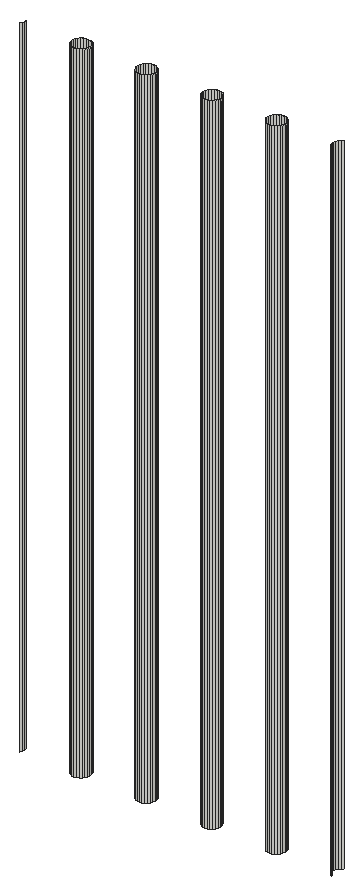
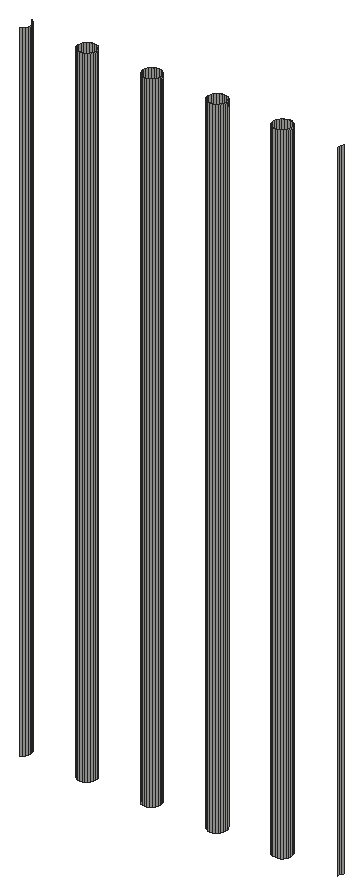
# SketchUp Ruby script. Lengths in inches.
U = 1.inch
M = Sketchup.active_model
def pt(a) = Geom::Point3d.new(a.map { |v| v * U })
def face(e, loops, mat)
  f = e.add_face(loops[0].map { |a| pt(a) })
  loops[1..].each { |l| e.add_face(l.map { |a| pt(a) }).erase! }
  f.material = f.back_material = mat if mat
  f
end
# faces: each face lists its corners as indices into pts; further lists are holes
def faces(e, pts, list, mat = nil) = list.each { |f| face(e, (f[0].is_a?(Array) ? f : [f]).map { |l| l.map { |i| pts[i] } }, mat) }
# xy, xz, yz: faces in a plane at the given z, y or x. An outline is a flat list of corners, or four numbers for a rectangle; further outlines are holes
def ring(l) = l.size == 4 ? [[l[0], l[1]], [l[2], l[1]], [l[2], l[3]], [l[0], l[3]]] : l.each_slice(2).to_a
def flat(e, list, mat, &to3) = list.each { |f| face(e, (f[0].is_a?(Array) ? f : [f]).map { |l| ring(l).map { |u, v| to3.(u, v) } }, mat) }
def xy(e, z, list, mat = nil) = flat(e, list, mat) { |x, y| [x, y, z] }
def xz(e, y, list, mat = nil) = flat(e, list, mat) { |x, z| [x, y, z] }
def yz(e, x, list, mat = nil) = flat(e, list, mat) { |y, z| [x, y, z] }
def lines(e, pts, list) = list.each { |a, b| e.add_line(pt(pts[a]), pt(pts[b])) }
# prism: a flat outline (further loops are holes) pulled along v
def prism(e, loops, v, mat = nil)
  f = face(e, loops, mat); d = Geom::Vector3d.new(v.map { |x| x * U })
  f.pushpull(f.normal.samedirection?(d) ? d.length : -d.length)
end
def box(e, o, s, mat = nil) = prism(e, [[o, [o[0] + s[0], o[1], o[2]], [o[0] + s[0], o[1] + s[1], o[2]], [o[0], o[1] + s[1], o[2]]]], [0, 0, s[2]], mat)
def at(x, y, z, deg = 0) = Geom::Transformation.translation(pt([x, y, z])) * Geom::Transformation.rotation(ORIGIN, Z_AXIS, deg.degrees)
def axes(o, x, y, z) = Geom::Transformation.new([*x, 0, *y, 0, *z, 0, *pt(o).to_a, 1])
def part(name) = M.definitions.add(name)
# library, detail: a bought-in or finely detailed component or shape, given as its bounding box
def library(name, o, s) = part(name).tap { |d| box(d.entities, o, s) }
def detail(e, o, s) = box(e.add_group.entities, o, s)
def put(e, d, t, mat = nil) = e.add_instance(d, t).tap { |i| i.material = mat if mat }
def group(e, t, mat = nil) = e.add_group.tap { |g| g.transformation = t; g.material = mat if mat }.entities
root = M.entities
xy(root,204.9375,[[448.33,135.31,448.12,135.34,447.92,135.42,447.75,135.55,447.625,135.72,447.54,135.91,447.52,136.12,447.54,136.33,447.625,136.53,447.75,136.7,447.92,136.83,448.12,136.91,448.33,136.93,448.54,136.91,448.74,136.83,448.9,136.7,449.03,136.53,449.11,136.33,449.14,136.12,449.11,135.91,449.03,135.72,448.9,135.55,448.74,135.42,448.54,135.34],[454.33,135.31,454.12,135.34,453.92,135.42,453.75,135.55,453.625,135.72,453.54,135.91,453.52,136.12,453.54,136.33,453.625,136.53,453.75,136.7,453.92,136.83,454.12,136.91,454.33,136.93,454.54,136.91,454.74,136.83,454.9,136.7,455.03,136.53,455.11,136.33,455.14,136.12,455.11,135.91,455.03,135.72,454.9,135.55,454.74,135.42,454.54,135.34],[460.33,135.31,460.12,135.34,459.92,135.42,459.75,135.55,459.625,135.72,459.54,135.91,459.52,136.12,459.54,136.33,459.625,136.53,459.75,136.7,459.92,136.83,460.12,136.91,460.33,136.93,460.54,136.91,460.74,136.83,460.9,136.7,461.03,136.53,461.11,136.33,461.14,136.12,461.11,135.91,461.03,135.72,460.9,135.55,460.74,135.42,460.54,135.34],[466.27,135.31,466.06,135.34,465.86,135.42,465.69,135.55,465.5625,135.72,465.48,135.91,465.45,136.12,465.48,136.33,465.5625,136.53,465.69,136.7,465.86,136.83,466.06,136.91,466.27,136.93,466.48,136.91,466.67,136.83,466.84,136.7,466.97,136.53,467.05,136.33,467.08,136.12,467.05,135.91,466.97,135.72,466.84,135.55,466.67,135.42,466.48,135.34]])
p = [[447.92,135.42,204.9375],[448.12,135.34,204.9375],[448.12,135.34,264.83],[447.92,135.42,264.83],[448.33,135.31,204.9375],[448.33,135.31,264.83],
  [448.54,135.34,204.9375],[448.54,135.34,264.83],[448.74,135.42,204.9375],[448.74,135.42,264.83],[453.92,135.42,204.9375],[454.12,135.34,204.9375],
  [454.12,135.34,264.83],[453.92,135.42,264.83],[454.33,135.31,204.9375],[454.33,135.31,264.83],[454.54,135.34,204.9375],[454.54,135.34,264.83],
  [454.74,135.42,204.9375],[454.74,135.42,264.83],[459.92,135.42,204.9375],[460.12,135.34,204.9375],[460.12,135.34,264.83],[459.92,135.42,264.83],
  [460.33,135.31,204.9375],[460.33,135.31,264.83],[460.54,135.34,204.9375],[460.54,135.34,264.83],[460.74,135.42,204.9375],[460.74,135.42,264.83],
  [465.86,135.42,204.9375],[466.06,135.34,204.9375],[466.06,135.34,264.83],[465.86,135.42,264.83],[466.27,135.31,204.9375],[466.27,135.31,264.83],
  [466.48,135.34,204.9375],[466.48,135.34,264.83],[466.67,135.42,204.9375],[466.67,135.42,264.83],[447.75,135.55,204.9375],[447.75,135.55,264.83],
  [448.9,135.55,204.9375],[448.9,135.55,264.83],[453.75,135.55,204.9375],[453.75,135.55,264.83],[454.9,135.55,204.9375],[454.9,135.55,264.83],
  [459.75,135.55,204.9375],[459.75,135.55,264.83],[460.9,135.55,204.9375],[460.9,135.55,264.83],[465.69,135.55,204.9375],[465.69,135.55,264.83],
  [466.84,135.55,204.9375],[466.84,135.55,264.83],[471.69,135.55,204.9375],[471.86,135.42,204.9375],[471.86,135.42,264.83],[471.69,135.55,264.83],
  [447.625,135.72,204.9375],[447.625,135.72,264.83],[449.03,135.72,204.9375],[449.03,135.72,264.83],[453.625,135.72,204.9375],[453.625,135.72,264.83],
  [455.03,135.72,204.9375],[455.03,135.72,264.83],[459.625,135.72,204.9375],[459.625,135.72,264.83],[461.03,135.72,204.9375],[461.03,135.72,264.83],
  [465.5625,135.72,204.9375],[465.5625,135.72,264.83],[466.97,135.72,204.9375],[466.97,135.72,264.83],[471.5625,135.72,204.9375],[471.5625,135.72,264.83],
  [443.03,135.72,204.9375],[443.11,135.91,204.9375],[443.11,135.91,264.83],[443.03,135.72,264.83],[447.54,135.91,204.9375],[447.54,135.91,264.83],
  [449.11,135.91,204.9375],[449.11,135.91,264.83],[453.54,135.91,204.9375],[453.54,135.91,264.83],[455.11,135.91,204.9375],[455.11,135.91,264.83],
  [459.54,135.91,204.9375],[459.54,135.91,264.83],[461.11,135.91,204.9375],[461.11,135.91,264.83],[465.48,135.91,204.9375],[465.48,135.91,264.83],
  [467.05,135.91,204.9375],[467.05,135.91,264.83],[471.48,135.91,204.9375],[471.48,135.91,264.83],[443.14,136.12,204.9375],[443.14,136.12,264.83],
  [447.52,136.12,204.9375],[447.52,136.12,264.83],[449.14,136.12,204.9375],[449.14,136.12,264.83],[453.52,136.12,204.9375],[453.52,136.12,264.83],
  [455.14,136.12,204.9375],[455.14,136.12,264.83],[459.52,136.12,204.9375],[459.52,136.12,264.83],[461.14,136.12,204.9375],[461.14,136.12,264.83],
  [465.45,136.12,204.9375],[465.45,136.12,264.83],[467.08,136.12,204.9375],[467.08,136.12,264.83],[471.45,136.12,204.9375],[471.45,136.12,264.83],
  [443.11,136.33,204.9375],[443.11,136.33,264.83],[447.54,136.33,204.9375],[447.54,136.33,264.83],[449.11,136.33,204.9375],[449.11,136.33,264.83],
  [453.54,136.33,204.9375],[453.54,136.33,264.83],[455.11,136.33,204.9375],[455.11,136.33,264.83],[459.54,136.33,204.9375],[459.54,136.33,264.83],
  [461.11,136.33,204.9375],[461.11,136.33,264.83],[465.48,136.33,204.9375],[465.48,136.33,264.83],[467.05,136.33,204.9375],[467.05,136.33,264.83],
  [471.48,136.33,204.9375],[471.48,136.33,264.83],[447.625,136.53,204.9375],[447.625,136.53,264.83],[449.03,136.53,204.9375],[449.03,136.53,264.83],
  [453.625,136.53,204.9375],[453.625,136.53,264.83],[455.03,136.53,204.9375],[455.03,136.53,264.83],[459.625,136.53,204.9375],[459.625,136.53,264.83],
  [461.03,136.53,204.9375],[461.03,136.53,264.83],[465.5625,136.53,204.9375],[465.5625,136.53,264.83],[466.97,136.53,204.9375],[466.97,136.53,264.83],
  [471.5625,136.53,204.9375],[471.5625,136.53,264.83],[447.75,136.7,204.9375],[447.75,136.7,264.83],[448.9,136.7,204.9375],[448.9,136.7,264.83],
  [453.75,136.7,204.9375],[453.75,136.7,264.83],[454.9,136.7,204.9375],[454.9,136.7,264.83],[459.75,136.7,204.9375],[459.75,136.7,264.83],
  [460.9,136.7,204.9375],[460.9,136.7,264.83],[465.69,136.7,204.9375],[465.69,136.7,264.83],[466.84,136.7,204.9375],[466.84,136.7,264.83],
  [471.69,136.7,204.9375],[471.69,136.7,264.83],[447.92,136.83,204.9375],[447.92,136.83,264.83],[448.74,136.83,204.9375],[448.74,136.83,264.83],
  [453.92,136.83,204.9375],[453.92,136.83,264.83],[454.74,136.83,204.9375],[454.74,136.83,264.83],[459.92,136.83,204.9375],[459.92,136.83,264.83],
  [460.74,136.83,204.9375],[460.74,136.83,264.83],[465.86,136.83,204.9375],[465.86,136.83,264.83],[466.67,136.83,204.9375],[466.67,136.83,264.83],
  [471.86,136.83,204.9375],[471.86,136.83,264.83],[448.12,136.91,204.9375],[448.12,136.91,264.83],[448.54,136.91,204.9375],[448.54,136.91,264.83],
  [454.12,136.91,204.9375],[454.12,136.91,264.83],[454.54,136.91,204.9375],[454.54,136.91,264.83],[460.12,136.91,204.9375],[460.12,136.91,264.83],
  [460.54,136.91,204.9375],[460.54,136.91,264.83],[466.06,136.91,204.9375],[466.06,136.91,264.83],[466.48,136.91,204.9375],[466.48,136.91,264.83],
  [448.33,136.93,204.9375],[448.33,136.93,264.83],[454.33,136.93,204.9375],[454.33,136.93,264.83],[460.33,136.93,204.9375],[460.33,136.93,264.83],
  [466.27,136.93,204.9375],[466.27,136.93,264.83],[466.27,136.12,264.83],[466.27,136.12,204.9375],[460.27,136.12,264.83],[460.27,136.12,204.9375],
  [454.27,136.12,264.83],[454.27,136.12,204.9375],[448.27,136.12,264.83],[448.27,136.12,204.9375]]
faces(root,p,[[0,1,2,3],[1,4,5,2],[4,6,7,5],[6,8,9,7],[10,11,12,13],[11,14,15,12],[14,16,17,15],[16,18,19,17],
  [20,21,22,23],[21,24,25,22],[24,26,27,25],[26,28,29,27],[30,31,32,33],[31,34,35,32],[34,36,37,35],[36,38,39,37],
  [40,0,3,41],[8,42,43,9],[44,10,13,45],[18,46,47,19],[48,20,23,49],[28,50,51,29],[52,30,33,53],[38,54,55,39],
  [56,57,58,59],[60,40,41,61],[42,62,63,43],[64,44,45,65],[46,66,67,47],[68,48,49,69],[50,70,71,51],[72,52,53,73],
  [54,74,75,55],[76,56,59,77],[78,79,80,81],[82,60,61,83],[62,84,85,63],[86,64,65,87],[66,88,89,67],[90,68,69,91],
  [70,92,93,71],[94,72,73,95],[74,96,97,75],[98,76,77,99],[79,100,101,80],[102,82,83,103],[84,104,105,85],[106,86,87,107],
  [88,108,109,89],[110,90,91,111],[92,112,113,93],[114,94,95,115],[96,116,117,97],[118,98,99,119],[100,120,121,101],[122,102,103,123],
  [104,124,125,105],[126,106,107,127],[108,128,129,109],[130,110,111,131],[112,132,133,113],[134,114,115,135],[116,136,137,117],[138,118,119,139],
  [140,122,123,141],[124,142,143,125],[144,126,127,145],[128,146,147,129],[148,130,131,149],[132,150,151,133],[152,134,135,153],[136,154,155,137],
  [156,138,139,157],[158,140,141,159],[142,160,161,143],[162,144,145,163],[146,164,165,147],[166,148,149,167],[150,168,169,151],[170,152,153,171],
  [154,172,173,155],[174,156,157,175],[176,158,159,177],[160,178,179,161],[180,162,163,181],[164,182,183,165],[184,166,167,185],[168,186,187,169],
  [188,170,171,189],[172,190,191,173],[192,174,175,193],[194,176,177,195],[178,196,197,179],[198,180,181,199],[182,200,201,183],[202,184,185,203],
  [186,204,205,187],[206,188,189,207],[190,208,209,191],[210,194,195,211],[196,210,211,197],[212,198,199,213],[200,212,213,201],[214,202,203,215],
  [204,214,215,205],[216,206,207,217],[208,216,217,209]])
lines(root,p,[[218,219],[220,221],[222,223],[224,225]])
